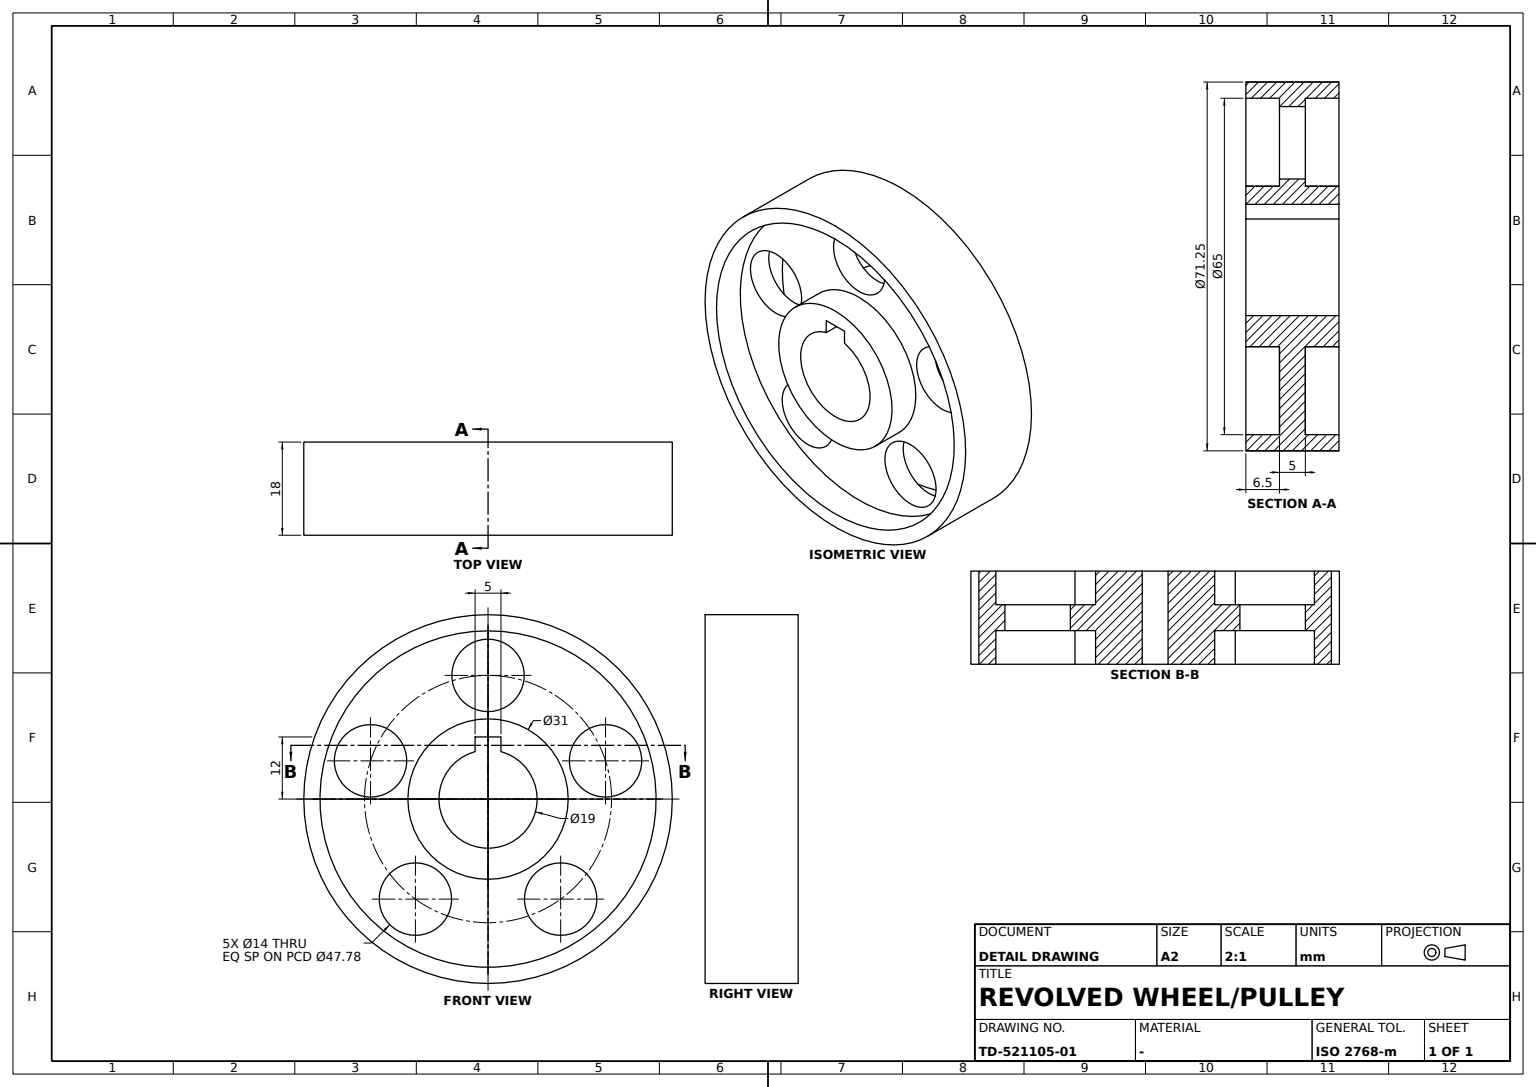
ISO-10303-21;
HEADER;
FILE_DESCRIPTION((''),'2;1');
FILE_NAME('','',(''),(''),'','','');
FILE_SCHEMA(('AUTOMOTIVE_DESIGN'));
ENDSEC;
DATA;
#1=APPLICATION_CONTEXT('');
#2=PRODUCT_CONTEXT('',#1,'mechanical');
#3=PRODUCT('','','',(#2));
#4=PRODUCT_DEFINITION_FORMATION('','',#3);
#5=PRODUCT_DEFINITION_CONTEXT('',#1,'design');
#6=PRODUCT_DEFINITION('','',#4,#5);
#7=PRODUCT_DEFINITION_SHAPE('','',#6);
#8=(LENGTH_UNIT()NAMED_UNIT(*)SI_UNIT(.MILLI.,.METRE.));
#9=(NAMED_UNIT(*)PLANE_ANGLE_UNIT()SI_UNIT($,.RADIAN.));
#10=(NAMED_UNIT(*)SI_UNIT($,.STERADIAN.)SOLID_ANGLE_UNIT());
#11=UNCERTAINTY_MEASURE_WITH_UNIT(LENGTH_MEASURE(0.005),#8,'distance_accuracy_value','');
#12=(GEOMETRIC_REPRESENTATION_CONTEXT(3)GLOBAL_UNCERTAINTY_ASSIGNED_CONTEXT((#11))GLOBAL_UNIT_ASSIGNED_CONTEXT((#8,#9,#10))REPRESENTATION_CONTEXT('',''));
#13=CARTESIAN_POINT('',(5.7,0.,32.5));
#14=VERTEX_POINT('',#13);
#15=CARTESIAN_POINT('',(5.7,0.,0.));
#16=DIRECTION('',(-1.,0.,0.));
#17=DIRECTION('',(0.,0.,1.));
#18=AXIS2_PLACEMENT_3D('',#15,#16,#17);
#19=CIRCLE('',#18,32.5);
#20=EDGE_CURVE('',#14,#14,#19,.T.);
#21=ORIENTED_EDGE('',*,*,#20,.F.);
#22=EDGE_LOOP('',(#21));
#23=FACE_BOUND('',#22,.T.);
#24=CARTESIAN_POINT('',(-0.8,0.,32.5));
#25=VERTEX_POINT('',#24);
#26=CARTESIAN_POINT('',(-0.8,0.,0.));
#27=AXIS2_PLACEMENT_3D('',#26,#16,#17);
#28=CIRCLE('',#27,32.5);
#29=EDGE_CURVE('',#25,#25,#28,.T.);
#30=ORIENTED_EDGE('',*,*,#29,.T.);
#31=EDGE_LOOP('',(#30));
#32=FACE_BOUND('',#31,.T.);
#33=CARTESIAN_POINT('',(-3.3,0.,0.));
#34=DIRECTION('',(0.,1.,0.));
#35=AXIS2_PLACEMENT_3D('',#33,#16,#34);
#36=CYLINDRICAL_SURFACE('',#35,32.5);
#37=ADVANCED_FACE('',(#23,#32),#36,.F.);
#38=CARTESIAN_POINT('',(-5.8,0.,30.89));
#39=VERTEX_POINT('',#38);
#40=CARTESIAN_POINT('',(-5.8,0.,23.89));
#41=AXIS2_PLACEMENT_3D('',#40,#16,#17);
#42=CIRCLE('',#41,7.);
#43=EDGE_CURVE('',#39,#39,#42,.T.);
#44=ORIENTED_EDGE('',*,*,#43,.F.);
#45=EDGE_LOOP('',(#44));
#46=FACE_BOUND('',#45,.T.);
#47=CARTESIAN_POINT('',(-5.8,14.04219,-12.327416));
#48=VERTEX_POINT('',#47);
#49=CARTESIAN_POINT('',(-5.8,14.04219,-19.327416));
#50=AXIS2_PLACEMENT_3D('',#49,#16,#17);
#51=CIRCLE('',#50,7.);
#52=EDGE_CURVE('',#48,#48,#51,.T.);
#53=ORIENTED_EDGE('',*,*,#52,.F.);
#54=EDGE_LOOP('',(#53));
#55=FACE_BOUND('',#54,.T.);
#56=CARTESIAN_POINT('',(-5.8,0.,32.5));
#57=VERTEX_POINT('',#56);
#58=CARTESIAN_POINT('',(-5.8,0.,0.));
#59=AXIS2_PLACEMENT_3D('',#58,#16,#17);
#60=CIRCLE('',#59,32.5);
#61=EDGE_CURVE('',#57,#57,#60,.T.);
#62=ORIENTED_EDGE('',*,*,#61,.T.);
#63=EDGE_LOOP('',(#62));
#64=FACE_BOUND('',#63,.T.);
#65=CARTESIAN_POINT('',(-5.8,-22.72074,14.382416));
#66=VERTEX_POINT('',#65);
#67=CARTESIAN_POINT('',(-5.8,-22.72074,7.382416));
#68=AXIS2_PLACEMENT_3D('',#67,#16,#17);
#69=CIRCLE('',#68,7.);
#70=EDGE_CURVE('',#66,#66,#69,.T.);
#71=ORIENTED_EDGE('',*,*,#70,.F.);
#72=EDGE_LOOP('',(#71));
#73=FACE_BOUND('',#72,.T.);
#74=CARTESIAN_POINT('',(-5.8,-14.04219,-12.327416));
#75=VERTEX_POINT('',#74);
#76=CARTESIAN_POINT('',(-5.8,-14.04219,-19.327416));
#77=AXIS2_PLACEMENT_3D('',#76,#16,#17);
#78=CIRCLE('',#77,7.);
#79=EDGE_CURVE('',#75,#75,#78,.T.);
#80=ORIENTED_EDGE('',*,*,#79,.F.);
#81=EDGE_LOOP('',(#80));
#82=FACE_BOUND('',#81,.T.);
#83=CARTESIAN_POINT('',(-5.8,22.72074,14.382416));
#84=VERTEX_POINT('',#83);
#85=CARTESIAN_POINT('',(-5.8,22.72074,7.382416));
#86=AXIS2_PLACEMENT_3D('',#85,#16,#17);
#87=CIRCLE('',#86,7.);
#88=EDGE_CURVE('',#84,#84,#87,.T.);
#89=ORIENTED_EDGE('',*,*,#88,.F.);
#90=EDGE_LOOP('',(#89));
#91=FACE_BOUND('',#90,.T.);
#92=CARTESIAN_POINT('',(-5.8,0.,15.5));
#93=VERTEX_POINT('',#92);
#94=CIRCLE('',#59,15.5);
#95=EDGE_CURVE('',#93,#93,#94,.T.);
#96=ORIENTED_EDGE('',*,*,#95,.F.);
#97=EDGE_LOOP('',(#96));
#98=FACE_BOUND('',#97,.T.);
#99=AXIS2_PLACEMENT_3D('',#56,#16,#34);
#100=PLANE('',#99);
#101=ADVANCED_FACE('',(#46,#55,#64,#73,#82,#91,#98),#100,.T.);
#102=CARTESIAN_POINT('',(-0.8,14.04219,-12.327416));
#103=VERTEX_POINT('',#102);
#104=CARTESIAN_POINT('',(-0.8,14.04219,-19.327416));
#105=AXIS2_PLACEMENT_3D('',#104,#16,#17);
#106=CIRCLE('',#105,7.);
#107=EDGE_CURVE('',#103,#103,#106,.T.);
#108=ORIENTED_EDGE('',*,*,#107,.F.);
#109=EDGE_LOOP('',(#108));
#110=FACE_BOUND('',#109,.T.);
#111=ORIENTED_EDGE('',*,*,#52,.T.);
#112=EDGE_LOOP('',(#111));
#113=FACE_BOUND('',#112,.T.);
#114=CARTESIAN_POINT('',(0.,14.04219,-19.327416));
#115=DIRECTION('',(1.,0.,0.));
#116=AXIS2_PLACEMENT_3D('',#114,#115,#34);
#117=CYLINDRICAL_SURFACE('',#116,7.);
#118=ADVANCED_FACE('',(#110,#113),#117,.F.);
#119=CARTESIAN_POINT('',(5.7,0.,35.625));
#120=VERTEX_POINT('',#119);
#121=CIRCLE('',#18,35.625);
#122=EDGE_CURVE('',#120,#120,#121,.T.);
#123=ORIENTED_EDGE('',*,*,#122,.T.);
#124=EDGE_LOOP('',(#123));
#125=FACE_BOUND('',#124,.T.);
#126=CARTESIAN_POINT('',(-12.3,0.,35.625));
#127=VERTEX_POINT('',#126);
#128=CARTESIAN_POINT('',(-12.3,0.,0.));
#129=AXIS2_PLACEMENT_3D('',#128,#16,#17);
#130=CIRCLE('',#129,35.625);
#131=EDGE_CURVE('',#127,#127,#130,.T.);
#132=ORIENTED_EDGE('',*,*,#131,.F.);
#133=EDGE_LOOP('',(#132));
#134=FACE_BOUND('',#133,.T.);
#135=CYLINDRICAL_SURFACE('',#35,35.625);
#136=ADVANCED_FACE('',(#125,#134),#135,.T.);
#137=CARTESIAN_POINT('',(-0.8,-14.04219,-12.327416));
#138=VERTEX_POINT('',#137);
#139=CARTESIAN_POINT('',(-0.8,-14.04219,-19.327416));
#140=AXIS2_PLACEMENT_3D('',#139,#16,#17);
#141=CIRCLE('',#140,7.);
#142=EDGE_CURVE('',#138,#138,#141,.T.);
#143=ORIENTED_EDGE('',*,*,#142,.F.);
#144=EDGE_LOOP('',(#143));
#145=FACE_BOUND('',#144,.T.);
#146=ORIENTED_EDGE('',*,*,#79,.T.);
#147=EDGE_LOOP('',(#146));
#148=FACE_BOUND('',#147,.T.);
#149=CARTESIAN_POINT('',(0.,-14.04219,-19.327416));
#150=AXIS2_PLACEMENT_3D('',#149,#115,#34);
#151=CYLINDRICAL_SURFACE('',#150,7.);
#152=ADVANCED_FACE('',(#145,#148),#151,.F.);
#153=ORIENTED_EDGE('',*,*,#122,.F.);
#154=EDGE_LOOP('',(#153));
#155=FACE_BOUND('',#154,.T.);
#156=ORIENTED_EDGE('',*,*,#20,.T.);
#157=EDGE_LOOP('',(#156));
#158=FACE_BOUND('',#157,.T.);
#159=AXIS2_PLACEMENT_3D('',#13,#16,#34);
#160=PLANE('',#159);
#161=ADVANCED_FACE('',(#155,#158),#160,.F.);
#162=ORIENTED_EDGE('',*,*,#61,.F.);
#163=EDGE_LOOP('',(#162));
#164=FACE_BOUND('',#163,.T.);
#165=CARTESIAN_POINT('',(-12.3,0.,32.5));
#166=VERTEX_POINT('',#165);
#167=CIRCLE('',#129,32.5);
#168=EDGE_CURVE('',#166,#166,#167,.T.);
#169=ORIENTED_EDGE('',*,*,#168,.T.);
#170=EDGE_LOOP('',(#169));
#171=FACE_BOUND('',#170,.T.);
#172=ADVANCED_FACE('',(#164,#171),#36,.F.);
#173=CARTESIAN_POINT('',(-0.8,0.,30.89));
#174=VERTEX_POINT('',#173);
#175=CARTESIAN_POINT('',(-0.8,0.,23.89));
#176=AXIS2_PLACEMENT_3D('',#175,#16,#17);
#177=CIRCLE('',#176,7.);
#178=EDGE_CURVE('',#174,#174,#177,.T.);
#179=ORIENTED_EDGE('',*,*,#178,.F.);
#180=EDGE_LOOP('',(#179));
#181=FACE_BOUND('',#180,.T.);
#182=ORIENTED_EDGE('',*,*,#43,.T.);
#183=EDGE_LOOP('',(#182));
#184=FACE_BOUND('',#183,.T.);
#185=CARTESIAN_POINT('',(0.,0.,23.89));
#186=AXIS2_PLACEMENT_3D('',#185,#115,#34);
#187=CYLINDRICAL_SURFACE('',#186,7.);
#188=ADVANCED_FACE('',(#181,#184),#187,.F.);
#189=CARTESIAN_POINT('',(-0.8,-22.72074,14.382416));
#190=VERTEX_POINT('',#189);
#191=CARTESIAN_POINT('',(-0.8,-22.72074,7.382416));
#192=AXIS2_PLACEMENT_3D('',#191,#16,#17);
#193=CIRCLE('',#192,7.);
#194=EDGE_CURVE('',#190,#190,#193,.T.);
#195=ORIENTED_EDGE('',*,*,#194,.F.);
#196=EDGE_LOOP('',(#195));
#197=FACE_BOUND('',#196,.T.);
#198=ORIENTED_EDGE('',*,*,#70,.T.);
#199=EDGE_LOOP('',(#198));
#200=FACE_BOUND('',#199,.T.);
#201=CARTESIAN_POINT('',(0.,-22.72074,7.382416));
#202=AXIS2_PLACEMENT_3D('',#201,#115,#34);
#203=CYLINDRICAL_SURFACE('',#202,7.);
#204=ADVANCED_FACE('',(#197,#200),#203,.F.);
#205=ORIENTED_EDGE('',*,*,#168,.F.);
#206=EDGE_LOOP('',(#205));
#207=FACE_BOUND('',#206,.T.);
#208=ORIENTED_EDGE('',*,*,#131,.T.);
#209=EDGE_LOOP('',(#208));
#210=FACE_BOUND('',#209,.T.);
#211=CARTESIAN_POINT('',(-12.3,0.,15.5));
#212=AXIS2_PLACEMENT_3D('',#211,#16,#34);
#213=PLANE('',#212);
#214=ADVANCED_FACE('',(#207,#210),#213,.T.);
#215=CARTESIAN_POINT('',(-12.3,2.5,9.165151));
#216=VERTEX_POINT('',#215);
#217=CARTESIAN_POINT('',(-12.3,-2.5,9.165151));
#218=VERTEX_POINT('',#217);
#219=CIRCLE('',#129,9.5);
#220=EDGE_CURVE('',#216,#218,#219,.T.);
#221=ORIENTED_EDGE('',*,*,#220,.T.);
#222=CARTESIAN_POINT('',(5.7,-2.5,9.165151));
#223=VERTEX_POINT('',#222);
#224=VECTOR('',#16,1000.);
#225=LINE('',#222,#224);
#226=EDGE_CURVE('',#223,#218,#225,.T.);
#227=ORIENTED_EDGE('',*,*,#226,.F.);
#228=CARTESIAN_POINT('',(5.7,2.5,9.165151));
#229=VERTEX_POINT('',#228);
#230=CIRCLE('',#18,9.5);
#231=EDGE_CURVE('',#229,#223,#230,.T.);
#232=ORIENTED_EDGE('',*,*,#231,.F.);
#233=LINE('',#228,#224);
#234=EDGE_CURVE('',#229,#216,#233,.T.);
#235=ORIENTED_EDGE('',*,*,#234,.T.);
#236=EDGE_LOOP('',(#221,#227,#232,#235));
#237=FACE_BOUND('',#236,.T.);
#238=CYLINDRICAL_SURFACE('',#35,9.5);
#239=ADVANCED_FACE('',(#237),#238,.F.);
#240=CARTESIAN_POINT('',(5.7,-2.5,12.));
#241=VERTEX_POINT('',#240);
#242=CARTESIAN_POINT('',(-12.3,-2.5,12.));
#243=VERTEX_POINT('',#242);
#244=CARTESIAN_POINT('',(0.,-2.5,12.));
#245=LINE('',#244,#224);
#246=EDGE_CURVE('',#241,#243,#245,.T.);
#247=ORIENTED_EDGE('',*,*,#246,.T.);
#248=CARTESIAN_POINT('',(-12.3,2.5,12.));
#249=VERTEX_POINT('',#248);
#250=CARTESIAN_POINT('',(-12.3,0.,12.));
#251=VECTOR('',#34,1000.);
#252=LINE('',#250,#251);
#253=EDGE_CURVE('',#243,#249,#252,.T.);
#254=ORIENTED_EDGE('',*,*,#253,.T.);
#255=CARTESIAN_POINT('',(5.7,2.5,12.));
#256=VERTEX_POINT('',#255);
#257=CARTESIAN_POINT('',(0.,2.5,12.));
#258=LINE('',#257,#224);
#259=EDGE_CURVE('',#256,#249,#258,.T.);
#260=ORIENTED_EDGE('',*,*,#259,.F.);
#261=CARTESIAN_POINT('',(5.7,0.,12.));
#262=LINE('',#261,#251);
#263=EDGE_CURVE('',#241,#256,#262,.T.);
#264=ORIENTED_EDGE('',*,*,#263,.F.);
#265=EDGE_LOOP('',(#247,#254,#260,#264));
#266=FACE_BOUND('',#265,.T.);
#267=AXIS2_PLACEMENT_3D('',#244,#17,#34);
#268=PLANE('',#267);
#269=ADVANCED_FACE('',(#266),#268,.F.);
#270=VERTEX_POINT('',#211);
#271=CIRCLE('',#129,15.5);
#272=EDGE_CURVE('',#270,#270,#271,.T.);
#273=ORIENTED_EDGE('',*,*,#272,.F.);
#274=EDGE_LOOP('',(#273));
#275=FACE_BOUND('',#274,.T.);
#276=ORIENTED_EDGE('',*,*,#95,.T.);
#277=EDGE_LOOP('',(#276));
#278=FACE_BOUND('',#277,.T.);
#279=CYLINDRICAL_SURFACE('',#35,15.5);
#280=ADVANCED_FACE('',(#275,#278),#279,.T.);
#281=ORIENTED_EDGE('',*,*,#29,.F.);
#282=EDGE_LOOP('',(#281));
#283=FACE_BOUND('',#282,.T.);
#284=CARTESIAN_POINT('',(-0.8,0.,15.5));
#285=VERTEX_POINT('',#284);
#286=CIRCLE('',#27,15.5);
#287=EDGE_CURVE('',#285,#285,#286,.T.);
#288=ORIENTED_EDGE('',*,*,#287,.T.);
#289=EDGE_LOOP('',(#288));
#290=FACE_BOUND('',#289,.T.);
#291=ORIENTED_EDGE('',*,*,#107,.T.);
#292=EDGE_LOOP('',(#291));
#293=FACE_BOUND('',#292,.T.);
#294=ORIENTED_EDGE('',*,*,#178,.T.);
#295=EDGE_LOOP('',(#294));
#296=FACE_BOUND('',#295,.T.);
#297=ORIENTED_EDGE('',*,*,#142,.T.);
#298=EDGE_LOOP('',(#297));
#299=FACE_BOUND('',#298,.T.);
#300=ORIENTED_EDGE('',*,*,#194,.T.);
#301=EDGE_LOOP('',(#300));
#302=FACE_BOUND('',#301,.T.);
#303=CARTESIAN_POINT('',(-0.8,22.72074,14.382416));
#304=VERTEX_POINT('',#303);
#305=CARTESIAN_POINT('',(-0.8,22.72074,7.382416));
#306=AXIS2_PLACEMENT_3D('',#305,#16,#17);
#307=CIRCLE('',#306,7.);
#308=EDGE_CURVE('',#304,#304,#307,.T.);
#309=ORIENTED_EDGE('',*,*,#308,.T.);
#310=EDGE_LOOP('',(#309));
#311=FACE_BOUND('',#310,.T.);
#312=AXIS2_PLACEMENT_3D('',#284,#16,#34);
#313=PLANE('',#312);
#314=ADVANCED_FACE('',(#283,#290,#293,#296,#299,#302,#311),#313,.F.);
#315=ORIENTED_EDGE('',*,*,#88,.T.);
#316=EDGE_LOOP('',(#315));
#317=FACE_BOUND('',#316,.T.);
#318=ORIENTED_EDGE('',*,*,#308,.F.);
#319=EDGE_LOOP('',(#318));
#320=FACE_BOUND('',#319,.T.);
#321=CARTESIAN_POINT('',(0.,22.72074,7.382416));
#322=AXIS2_PLACEMENT_3D('',#321,#115,#34);
#323=CYLINDRICAL_SURFACE('',#322,7.);
#324=ADVANCED_FACE('',(#317,#320),#323,.F.);
#325=CARTESIAN_POINT('',(5.7,2.5,32.5));
#326=VECTOR('',#17,1000.);
#327=LINE('',#325,#326);
#328=EDGE_CURVE('',#229,#256,#327,.T.);
#329=ORIENTED_EDGE('',*,*,#328,.F.);
#330=ORIENTED_EDGE('',*,*,#231,.T.);
#331=CARTESIAN_POINT('',(5.7,-2.5,32.5));
#332=DIRECTION('',(0.,0.,-1.));
#333=VECTOR('',#332,1000.);
#334=LINE('',#331,#333);
#335=EDGE_CURVE('',#241,#223,#334,.T.);
#336=ORIENTED_EDGE('',*,*,#335,.F.);
#337=ORIENTED_EDGE('',*,*,#263,.T.);
#338=EDGE_LOOP('',(#329,#330,#336,#337));
#339=FACE_BOUND('',#338,.T.);
#340=CARTESIAN_POINT('',(5.7,0.,15.5));
#341=VERTEX_POINT('',#340);
#342=CIRCLE('',#18,15.5);
#343=EDGE_CURVE('',#341,#341,#342,.T.);
#344=ORIENTED_EDGE('',*,*,#343,.F.);
#345=EDGE_LOOP('',(#344));
#346=FACE_BOUND('',#345,.T.);
#347=ADVANCED_FACE('',(#339,#346),#160,.F.);
#348=CARTESIAN_POINT('',(-12.3,-2.5,15.5));
#349=LINE('',#348,#333);
#350=EDGE_CURVE('',#243,#218,#349,.T.);
#351=ORIENTED_EDGE('',*,*,#350,.F.);
#352=ORIENTED_EDGE('',*,*,#246,.F.);
#353=ORIENTED_EDGE('',*,*,#335,.T.);
#354=ORIENTED_EDGE('',*,*,#226,.T.);
#355=EDGE_LOOP('',(#351,#352,#353,#354));
#356=FACE_BOUND('',#355,.T.);
#357=AXIS2_PLACEMENT_3D('',#244,#34,#332);
#358=PLANE('',#357);
#359=ADVANCED_FACE('',(#356),#358,.T.);
#360=ORIENTED_EDGE('',*,*,#234,.F.);
#361=ORIENTED_EDGE('',*,*,#328,.T.);
#362=ORIENTED_EDGE('',*,*,#259,.T.);
#363=CARTESIAN_POINT('',(-12.3,2.5,15.5));
#364=LINE('',#363,#326);
#365=EDGE_CURVE('',#216,#249,#364,.T.);
#366=ORIENTED_EDGE('',*,*,#365,.F.);
#367=EDGE_LOOP('',(#360,#361,#362,#366));
#368=FACE_BOUND('',#367,.T.);
#369=CARTESIAN_POINT('',(0.,2.5,9.165151));
#370=DIRECTION('',(0.,-1.,0.));
#371=AXIS2_PLACEMENT_3D('',#369,#370,#17);
#372=PLANE('',#371);
#373=ADVANCED_FACE('',(#368),#372,.T.);
#374=ORIENTED_EDGE('',*,*,#272,.T.);
#375=EDGE_LOOP('',(#374));
#376=FACE_BOUND('',#375,.T.);
#377=ORIENTED_EDGE('',*,*,#365,.T.);
#378=ORIENTED_EDGE('',*,*,#253,.F.);
#379=ORIENTED_EDGE('',*,*,#350,.T.);
#380=ORIENTED_EDGE('',*,*,#220,.F.);
#381=EDGE_LOOP('',(#377,#378,#379,#380));
#382=FACE_BOUND('',#381,.T.);
#383=ADVANCED_FACE('',(#376,#382),#213,.T.);
#384=ORIENTED_EDGE('',*,*,#343,.T.);
#385=EDGE_LOOP('',(#384));
#386=FACE_BOUND('',#385,.T.);
#387=ORIENTED_EDGE('',*,*,#287,.F.);
#388=EDGE_LOOP('',(#387));
#389=FACE_BOUND('',#388,.T.);
#390=ADVANCED_FACE('',(#386,#389),#279,.T.);
#391=CLOSED_SHELL('',(#37,#101,#118,#136,#152,#161,#172,#188,#204,#214,#239,#269,#280,#314,#324,#347,#359,#373,#383,#390));
#392=MANIFOLD_SOLID_BREP('',#391);
#393=ADVANCED_BREP_SHAPE_REPRESENTATION('',(#392),#12);
#394=SHAPE_DEFINITION_REPRESENTATION(#7,#393);
ENDSEC;
END-ISO-10303-21;
